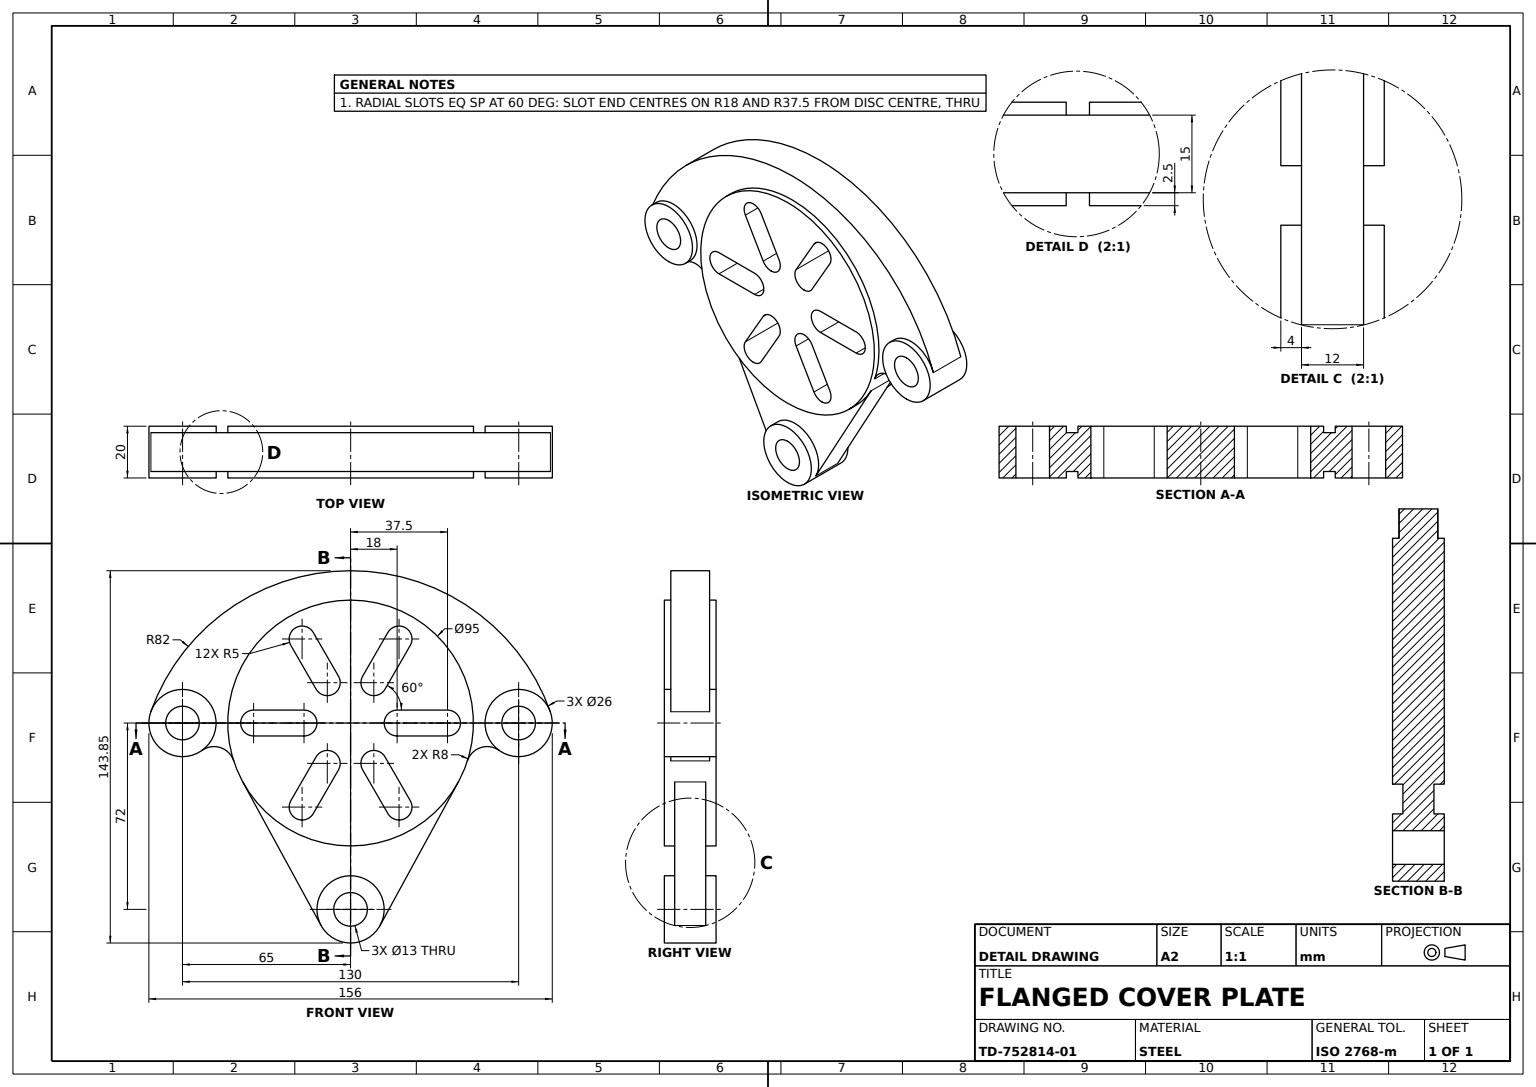
solid
v1 (-14.4198729811,0,-34.9759526419)
v2 (-14.4198729811,20,-34.9759526419)
e1 v1 v2 LINE
v3 (-23.0801270189,20,-29.9759526419)
e2 v2 v3 CIRCLE(AX(P(-18.75,20,-32.4759526419),D(0,1,0),D(0,0,1)),5)
v4 (-23.0801270189,0,-29.9759526419)
e3 v4 v3 LINE
e4 v1 v4 CIRCLE(AX(P(-18.75,0,-32.4759526419),D(0,1,0),D(0,0,1)),5)
face CYL(AX(P(-18.75,0,-32.4759526419),D(0,1,0),D(0,0,1)),5) rev [e1 e2 -e3 -e4]
v5 (9,0,-10.5884572681)
v6 (9,20,-10.5884572681)
e5 v5 v6 LINE
v7 (4.6698729811,0,-18.0884572681)
e6 v7 v5 CIRCLE(AX(P(9,0,-15.5884572681),D(0,1,0),D(0,0,1)),5)
v8 (4.6698729811,20,-18.0884572681)
e7 v7 v8 LINE
e8 v8 v6 CIRCLE(AX(P(9,20,-15.5884572681),D(0,1,0),D(0,0,1)),5)
face CYL(AX(P(9,0,-15.5884572681),D(0,1,0),D(0,0,1)),5) rev [-e5 -e6 e7 e8]
v9 (77.2463768116,2.5,-4.3619095576)
v10 (0,2.5,-58.8483261944)
e9 v9 v10 CIRCLE(AX(P(0,2.5,23.1516738056),D(0,1,0),D(0,0,-1)),82)
v11 (0,17.5,-58.8483261944)
e10 v11 v10 LINE
v12 (77.2463768116,17.5,-4.3619095576)
e11 v12 v11 CIRCLE(AX(P(0,17.5,23.1516738056),D(0,1,0),D(0,0,-1)),82)
e12 v12 v9 LINE
face CYL(AX(P(0,17.5,23.1516738056),D(0,-1,0),D(0,0,-1)),82) [e9 -e10 -e11 e12]
v13 (13.3301270189,0,13.0884572681)
v14 (13.3301270189,20,13.0884572681)
e13 v13 v14 LINE
v15 (23.0801270189,0,29.9759526419)
e14 v13 v15 LINE
v16 (23.0801270189,20,29.9759526419)
e15 v15 v16 LINE
e16 v14 v16 LINE
face PLANE(AX(P(4.3301270189,0,-2.5),D(-0.8660254038,0,0.5),D(0.5,0,0.8660254038))) [-e13 e14 e15 -e16]
v17 (65,20,6.5)
v18 (65,0,6.5)
e17 v17 v18 LINE
v19 (65,20,-6.5)
e18 v17 v19 CIRCLE(AX(P(65,20,0),D(0,1,0),D(0,0,1)),6.5)
v20 (65,0,-6.5)
e19 v19 v20 LINE
e20 v18 v20 CIRCLE(AX(P(65,0,0),D(0,1,0),D(0,0,1)),6.5)
face CYL(AX(P(65,20,0),D(0,-1,0),D(0,0,-1)),6.5) rev [-e17 e18 e19 -e20]
v21 (-13.3301270189,20,-13.0884572681)
e21 v21 v3 LINE
v22 (-13.3301270189,0,-13.0884572681)
e22 v22 v21 LINE
e23 v22 v4 LINE
face PLANE(AX(P(-4.3301270189,0,2.5),D(0.8660254038,0,-0.5),D(-0.5,0,-0.8660254038))) [-e21 -e22 e23 e3]
v23 (-52.8019230769,17.5,9.0940609388)
v24 (-52.8019230769,2.5,9.0940609388)
e24 v23 v24 LINE
v25 (-45.1908350658,2.5,14.6300521548)
e25 v24 v25 CIRCLE(AX(P(-52.8019230769,2.5,17.0940609388),D(0,-1,0),D(0,0,-1)),8)
v26 (-45.1908350658,17.5,14.6300521548)
e26 v26 v25 LINE
e27 v23 v26 CIRCLE(AX(P(-52.8019230769,17.5,17.0940609388),D(0,-1,0),D(0,0,-1)),8)
face CYL(AX(P(-52.8019230769,17.5,17.0940609388),D(0,-1,0),D(0,0,-1)),8) rev [e24 e25 -e26 -e27]
v27 (0,16,59)
v28 (11.4104111512,16,78.2291666667)
e28 v27 v28 CIRCLE(AX(P(0,16,72),D(0,-1,0),D(0,0,1)),13)
v29 (41.6918868985,16,22.7604166667)
e29 v28 v29 LINE
v30 (0,16,47.5)
e30 v29 v30 CIRCLE(AX(P(0,16,0),D(0,-1,0),D(0,0,1)),47.5)
v31 (-41.6918868985,16,22.7604166667)
e31 v30 v31 CIRCLE(AX(P(0,16,0),D(0,-1,0),D(0,0,1)),47.5)
v32 (-11.4104111512,16,78.2291666667)
e32 v31 v32 LINE
e33 v32 v27 CIRCLE(AX(P(0,16,72),D(0,-1,0),D(0,0,1)),13)
face PLANE(AX(P(0,16,0),D(0,1,0),D(0,0,1))) [e28 e29 e30 e31 e32 e33]
v33 (18,0,5)
v34 (37.5,0,5)
e34 v33 v34 LINE
v35 (18,20,5)
e35 v33 v35 LINE
v36 (37.5,20,5)
e36 v35 v36 LINE
e37 v34 v36 LINE
face PLANE(AX(P(0,0,5),D(0,0,1),D(1,0,0))) rev [-e34 e35 e36 -e37]
v37 (-57.4488095238,17.5,10.582037724)
v38 (-57.4488095238,2.5,10.582037724)
e38 v37 v38 LINE
e39 v38 v24 CIRCLE(AX(P(-52.8019230769,2.5,17.0940609388),D(0,-1,0),D(0,0,-1)),8)
e40 v37 v23 CIRCLE(AX(P(-52.8019230769,17.5,17.0940609388),D(0,-1,0),D(0,0,-1)),8)
face CYL(AX(P(-52.8019230769,17.5,17.0940609388),D(0,-1,0),D(0,0,-1)),8) rev [e38 e39 -e24 -e40]
v39 (-65,20,-6.5)
v40 (-65,0,-6.5)
e41 v39 v40 LINE
v41 (-65,0,6.5)
e42 v41 v40 CIRCLE(AX(P(-65,0,0),D(0,1,0),D(0,0,1)),6.5)
v42 (-65,20,6.5)
e43 v42 v41 LINE
e44 v42 v39 CIRCLE(AX(P(-65,20,0),D(0,1,0),D(0,0,1)),6.5)
face CYL(AX(P(-65,20,0),D(0,-1,0),D(0,0,-1)),6.5) rev [e41 -e42 -e43 e44]
v43 (4.6698729811,20,18.0884572681)
e45 v14 v43 CIRCLE(AX(P(9,20,15.5884572681),D(0,1,0),D(0,0,1)),5)
v44 (4.6698729811,0,18.0884572681)
e46 v44 v43 LINE
e47 v13 v44 CIRCLE(AX(P(9,0,15.5884572681),D(0,1,0),D(0,0,1)),5)
face CYL(AX(P(9,0,15.5884572681),D(0,1,0),D(0,0,1)),5) rev [e13 e45 -e46 -e47]
v45 (18,0,-5)
e48 v45 v33 CIRCLE(AX(P(18,0,0),D(0,1,0),D(0,0,1)),5)
v46 (18,20,-5)
e49 v45 v46 LINE
e50 v46 v35 CIRCLE(AX(P(18,20,0),D(0,1,0),D(0,0,1)),5)
face CYL(AX(P(18,0,0),D(0,1,0),D(0,0,1)),5) rev [-e48 e49 e50 -e35]
v47 (-4.6698729811,0,18.0884572681)
v48 (-13.3301270189,0,13.0884572681)
e51 v47 v48 CIRCLE(AX(P(-9,0,15.5884572681),D(0,1,0),D(0,0,1)),5)
v49 (-4.6698729811,20,18.0884572681)
e52 v47 v49 LINE
v50 (-13.3301270189,20,13.0884572681)
e53 v49 v50 CIRCLE(AX(P(-9,20,15.5884572681),D(0,1,0),D(0,0,1)),5)
e54 v48 v50 LINE
face CYL(AX(P(-9,0,15.5884572681),D(0,1,0),D(0,0,1)),5) rev [-e51 e52 e53 -e54]
v51 (65,17.5,-13)
e55 v12 v51 CIRCLE(AX(P(65,17.5,0),D(0,1,0),D(0,0,-1)),13)
v52 (65,20,-13)
e56 v52 v51 LINE
v53 (65,20,13)
e57 v53 v52 CIRCLE(AX(P(65,20,0),D(0,1,0),D(0,0,1)),13)
v54 (65,0,13)
e58 v53 v54 LINE
v55 (65,0,-13)
e59 v54 v55 CIRCLE(AX(P(65,0,0),D(0,1,0),D(0,0,1)),13)
v56 (65,2.5,-13)
e60 v56 v55 LINE
e61 v9 v56 CIRCLE(AX(P(65,2.5,0),D(0,1,0),D(0,0,-1)),13)
face CYL(AX(P(65,17.5,0),D(0,-1,0),D(0,0,-1)),13) [e55 -e56 -e57 e58 e59 -e60 -e61 -e12]
e62 v52 v53 CIRCLE(AX(P(65,20,0),D(0,1,0),D(0,0,1)),13)
v57 (57.4488095238,17.5,10.582037724)
e63 v51 v57 CIRCLE(AX(P(65,17.5,0),D(0,1,0),D(0,0,-1)),13)
v58 (57.4488095238,2.5,10.582037724)
e64 v57 v58 LINE
e65 v56 v58 CIRCLE(AX(P(65,2.5,0),D(0,1,0),D(0,0,-1)),13)
e66 v55 v54 CIRCLE(AX(P(65,0,0),D(0,1,0),D(0,0,1)),13)
face CYL(AX(P(65,17.5,0),D(0,-1,0),D(0,0,-1)),13) [-e58 -e62 e56 e63 e64 -e65 e60 e66]
v59 (0,4,59)
v60 (11.4104111512,4,78.2291666667)
e67 v59 v60 CIRCLE(AX(P(0,4,72),D(0,-1,0),D(0,0,1)),13)
v61 (-11.4104111512,4,78.2291666667)
e68 v61 v59 CIRCLE(AX(P(0,4,72),D(0,-1,0),D(0,0,1)),13)
v62 (-41.6918868985,4,22.7604166667)
e69 v62 v61 LINE
v63 (0,4,47.5)
e70 v63 v62 CIRCLE(AX(P(0,4,0),D(0,-1,0),D(0,0,1)),47.5)
v64 (41.6918868985,4,22.7604166667)
e71 v64 v63 CIRCLE(AX(P(0,4,0),D(0,-1,0),D(0,0,1)),47.5)
e72 v60 v64 LINE
face PLANE(AX(P(0,4,0),D(0,1,0),D(0,0,1))) rev [-e67 -e68 -e69 -e70 -e71 -e72]
v65 (13.3301270189,20,-13.0884572681)
e73 v6 v65 CIRCLE(AX(P(9,20,-15.5884572681),D(0,1,0),D(0,0,1)),5)
v66 (13.3301270189,0,-13.0884572681)
e74 v66 v65 LINE
e75 v5 v66 CIRCLE(AX(P(9,0,-15.5884572681),D(0,1,0),D(0,0,1)),5)
face CYL(AX(P(9,0,-15.5884572681),D(0,1,0),D(0,0,1)),5) rev [e73 -e74 -e75 e5]
v67 (-14.4198729811,20,34.9759526419)
e76 v49 v67 LINE
v68 (-14.4198729811,0,34.9759526419)
e77 v47 v68 LINE
e78 v68 v67 LINE
face PLANE(AX(P(4.3301270189,0,2.5),D(-0.8660254038,0,-0.5),D(-0.5,0,0.8660254038))) [-e76 -e52 e77 e78]
e79 v29 v64 LINE
e80 v28 v60 LINE
face PLANE(AX(P(41.6918868985,16,22.7604166667),D(-0.8777239347,0,-0.4791666667),D(-0.4791666667,0,0.8777239347))) rev [-e79 -e29 e80 e72]
e81 v19 v17 CIRCLE(AX(P(65,20,0),D(0,1,0),D(0,0,1)),6.5)
face PLANE(AX(P(65,20,0),D(0,1,0),D(0,0,1))) [e62 e57] [-e18 -e81]
v69 (-18.75,20,37.4759526419)
e82 v69 v67 CIRCLE(AX(P(-18.75,20,32.4759526419),D(0,1,0),D(0,0,1)),5)
v70 (-18.75,0,37.4759526419)
e83 v70 v68 CIRCLE(AX(P(-18.75,0,32.4759526419),D(0,1,0),D(0,0,1)),5)
e84 v70 v69 LINE
face CYL(AX(P(-18.75,0,32.4759526419),D(0,1,0),D(0,0,1)),5) rev [e82 -e78 -e83 e84]
v71 (0,20,85)
v72 (0,20,59)
e85 v71 v72 CIRCLE(AX(P(0,20,72),D(0,1,0),D(0,0,1)),13)
e86 v72 v71 CIRCLE(AX(P(0,20,72),D(0,1,0),D(0,0,1)),13)
v73 (0,20,65.5)
v74 (0,20,78.5)
e87 v73 v74 CIRCLE(AX(P(0,20,72),D(0,1,0),D(0,0,1)),6.5)
e88 v74 v73 CIRCLE(AX(P(0,20,72),D(0,1,0),D(0,0,1)),6.5)
face PLANE(AX(P(0,20,72),D(0,1,0),D(0,0,1))) [e85 e86] [-e87 -e88]
v75 (0,0,85)
v76 (0,0,59)
e89 v75 v76 CIRCLE(AX(P(0,0,72),D(0,1,0),D(0,0,1)),13)
e90 v76 v75 CIRCLE(AX(P(0,0,72),D(0,1,0),D(0,0,1)),13)
v77 (0,0,78.5)
v78 (0,0,65.5)
e91 v77 v78 CIRCLE(AX(P(0,0,72),D(0,1,0),D(0,0,1)),6.5)
e92 v78 v77 CIRCLE(AX(P(0,0,72),D(0,1,0),D(0,0,1)),6.5)
face PLANE(AX(P(0,0,72),D(0,1,0),D(0,0,1))) rev [-e89 -e90] [e91 e92]
v79 (23.0801270189,0,-29.9759526419)
v80 (14.4198729811,0,-34.9759526419)
e93 v79 v80 CIRCLE(AX(P(18.75,0,-32.4759526419),D(0,1,0),D(0,0,1)),5)
v81 (23.0801270189,20,-29.9759526419)
e94 v79 v81 LINE
v82 (14.4198729811,20,-34.9759526419)
e95 v81 v82 CIRCLE(AX(P(18.75,20,-32.4759526419),D(0,1,0),D(0,0,1)),5)
e96 v80 v82 LINE
face CYL(AX(P(18.75,0,-32.4759526419),D(0,1,0),D(0,0,1)),5) rev [-e93 e94 e95 -e96]
e97 v7 v80 LINE
e98 v8 v82 LINE
face PLANE(AX(P(-4.3301270189,0,-2.5),D(0.8660254038,0,0.5),D(0.5,0,-0.8660254038))) [e97 e96 -e98 -e7]
v83 (-23.0801270189,0,29.9759526419)
v84 (-23.0801270189,20,29.9759526419)
e99 v83 v84 LINE
e100 v84 v69 CIRCLE(AX(P(-18.75,20,32.4759526419),D(0,1,0),D(0,0,1)),5)
e101 v83 v70 CIRCLE(AX(P(-18.75,0,32.4759526419),D(0,1,0),D(0,0,1)),5)
face CYL(AX(P(-18.75,0,32.4759526419),D(0,1,0),D(0,0,1)),5) rev [e99 e100 -e84 -e101]
e102 v78 v73 LINE
e103 v77 v74 LINE
face CYL(AX(P(0,0,72),D(0,1,0),D(0,0,1)),6.5) rev [e102 e87 -e103 -e92]
v85 (-77.2463768116,17.5,-4.3619095576)
e104 v11 v85 CIRCLE(AX(P(0,17.5,23.1516738056),D(0,1,0),D(0,0,-1)),82)
v86 (-65,17.5,-13)
e105 v86 v85 CIRCLE(AX(P(-65,17.5,0),D(0,1,0),D(0,0,-1)),13)
e106 v37 v86 CIRCLE(AX(P(-65,17.5,0),D(0,1,0),D(0,0,-1)),13)
v87 (0,17.5,-47.5)
e107 v26 v87 CIRCLE(AX(P(0,17.5,0),D(0,-1,0),D(0,0,-1)),47.5)
v88 (45.1908350658,17.5,14.6300521548)
e108 v87 v88 CIRCLE(AX(P(0,17.5,0),D(0,-1,0),D(0,0,-1)),47.5)
v89 (52.8019230769,17.5,9.0940609388)
e109 v88 v89 CIRCLE(AX(P(52.8019230769,17.5,17.0940609388),D(0,-1,0),D(0,0,-1)),8)
e110 v89 v57 CIRCLE(AX(P(52.8019230769,17.5,17.0940609388),D(0,-1,0),D(0,0,-1)),8)
face PLANE(AX(P(32.5,17.5,11.5758369028),D(0,-1,0),D(0,0,-1))) rev [-e63 -e55 e11 e104 -e105 -e106 e40 e27 e107 e108 e109 e110]
v90 (-9,20,-10.5884572681)
v91 (-4.6698729811,20,-18.0884572681)
e111 v90 v91 CIRCLE(AX(P(-9,20,-15.5884572681),D(0,1,0),D(0,0,1)),5)
v92 (-4.6698729811,0,-18.0884572681)
e112 v92 v91 LINE
v93 (-9,0,-10.5884572681)
e113 v93 v92 CIRCLE(AX(P(-9,0,-15.5884572681),D(0,1,0),D(0,0,1)),5)
e114 v93 v90 LINE
face CYL(AX(P(-9,0,-15.5884572681),D(0,1,0),D(0,0,1)),5) rev [e111 -e112 -e113 e114]
v94 (18.75,0,37.4759526419)
v95 (18.75,20,37.4759526419)
e115 v94 v95 LINE
e116 v95 v16 CIRCLE(AX(P(18.75,20,32.4759526419),D(0,1,0),D(0,0,1)),5)
e117 v94 v15 CIRCLE(AX(P(18.75,0,32.4759526419),D(0,1,0),D(0,0,1)),5)
face CYL(AX(P(18.75,0,32.4759526419),D(0,1,0),D(0,0,1)),5) rev [e115 e116 -e15 -e117]
v96 (52.8019230769,2.5,9.0940609388)
e118 v89 v96 LINE
e119 v96 v58 CIRCLE(AX(P(52.8019230769,2.5,17.0940609388),D(0,-1,0),D(0,0,-1)),8)
face CYL(AX(P(52.8019230769,17.5,17.0940609388),D(0,-1,0),D(0,0,-1)),8) rev [e118 e119 -e64 -e110]
v97 (14.4198729811,0,34.9759526419)
v98 (14.4198729811,20,34.9759526419)
e120 v97 v98 LINE
e121 v98 v95 CIRCLE(AX(P(18.75,20,32.4759526419),D(0,1,0),D(0,0,1)),5)
e122 v97 v94 CIRCLE(AX(P(18.75,0,32.4759526419),D(0,1,0),D(0,0,1)),5)
face CYL(AX(P(18.75,0,32.4759526419),D(0,1,0),D(0,0,1)),5) rev [e120 e121 -e115 -e122]
v99 (-18,0,5)
v100 (-18,20,5)
e123 v99 v100 LINE
v101 (-18,20,-5)
e124 v100 v101 CIRCLE(AX(P(-18,20,0),D(0,1,0),D(0,0,1)),5)
v102 (-18,0,-5)
e125 v102 v101 LINE
e126 v99 v102 CIRCLE(AX(P(-18,0,0),D(0,1,0),D(0,0,1)),5)
face CYL(AX(P(-18,0,0),D(0,1,0),D(0,0,1)),5) rev [e123 e124 -e125 -e126]
e127 v31 v62 LINE
e128 v32 v61 LINE
face PLANE(AX(P(-41.6918868985,16,22.7604166667),D(0.8777239347,0,-0.4791666667),D(-0.4791666667,0,-0.8777239347))) rev [e127 e69 -e128 -e32]
e129 v50 v84 LINE
e130 v48 v83 LINE
face PLANE(AX(P(-4.3301270189,0,-2.5),D(-0.8660254038,0,-0.5),D(-0.5,0,0.8660254038))) rev [e129 -e99 -e130 e54]
v103 (37.5,20,-5)
e131 v46 v103 LINE
e132 v36 v103 CIRCLE(AX(P(37.5,20,0),D(0,1,0),D(0,0,1)),5)
v104 (0,20,47.5)
v105 (0,20,-47.5)
e133 v104 v105 CIRCLE(AX(P(0,20,0),D(0,1,0),D(0,0,1)),47.5)
e134 v105 v104 CIRCLE(AX(P(0,20,0),D(0,1,0),D(0,0,1)),47.5)
e135 v65 v81 LINE
e136 v21 v90 CIRCLE(AX(P(-9,20,-15.5884572681),D(0,1,0),D(0,0,1)),5)
e137 v91 v2 LINE
v106 (-37.5,20,5)
e138 v100 v106 LINE
v107 (-37.5,20,-5)
e139 v107 v106 CIRCLE(AX(P(-37.5,20,0),D(0,1,0),D(0,0,1)),5)
e140 v101 v107 LINE
e141 v43 v98 LINE
face PLANE(AX(P(0,20,0),D(0,1,0),D(0,0,1))) [e131 -e132 -e36 -e50] [e133 e134] [-e73 -e8 e98 -e95 -e135] [-e100 -e129 -e53 e76 -e82] [-e136 e21 -e2 -e137 -e111] [-e124 e138 -e139 -e140] [-e121 -e141 -e45 e16 -e116]
e142 v20 v18 CIRCLE(AX(P(65,0,0),D(0,1,0),D(0,0,1)),6.5)
face PLANE(AX(P(65,0,0),D(0,1,0),D(0,0,1))) rev [-e59 -e66] [e20 e142]
e143 v72 v27 LINE
e144 v71 v75 LINE
e145 v59 v76 LINE
face CYL(AX(P(0,16,72),D(0,-1,0),D(0,0,-1)),13) [-e28 -e143 -e85 e144 e89 -e145 e67 -e80]
v108 (37.5,0,-5)
e146 v45 v108 LINE
e147 v108 v103 LINE
face PLANE(AX(P(0,0,-5),D(0,0,1),D(1,0,0))) [e146 e147 -e131 -e49]
v109 (-77.2463768116,2.5,-4.3619095576)
e148 v10 v109 CIRCLE(AX(P(0,2.5,23.1516738056),D(0,1,0),D(0,0,-1)),82)
v110 (45.1908350658,2.5,14.6300521548)
e149 v110 v96 CIRCLE(AX(P(52.8019230769,2.5,17.0940609388),D(0,-1,0),D(0,0,-1)),8)
v111 (0,2.5,-47.5)
e150 v111 v110 CIRCLE(AX(P(0,2.5,0),D(0,-1,0),D(0,0,-1)),47.5)
e151 v25 v111 CIRCLE(AX(P(0,2.5,0),D(0,-1,0),D(0,0,-1)),47.5)
v112 (-65,2.5,-13)
e152 v38 v112 CIRCLE(AX(P(-65,2.5,0),D(0,1,0),D(0,0,-1)),13)
e153 v112 v109 CIRCLE(AX(P(-65,2.5,0),D(0,1,0),D(0,0,-1)),13)
face PLANE(AX(P(32.5,2.5,11.5758369028),D(0,-1,0),D(0,0,-1))) [-e148 -e9 e61 e65 -e119 -e149 -e150 -e151 -e25 -e39 e152 e153]
v113 (-65,20,-13)
v114 (-65,20,13)
e154 v113 v114 CIRCLE(AX(P(-65,20,0),D(0,1,0),D(0,0,1)),13)
e155 v113 v86 LINE
e156 v85 v109 LINE
v115 (-65,0,-13)
e157 v112 v115 LINE
v116 (-65,0,13)
e158 v115 v116 CIRCLE(AX(P(-65,0,0),D(0,1,0),D(0,0,1)),13)
e159 v114 v116 LINE
face CYL(AX(P(-65,17.5,0),D(0,-1,0),D(0,0,-1)),13) [-e154 e155 e105 e156 -e153 e157 e158 -e159]
face CYL(AX(P(0,17.5,23.1516738056),D(0,-1,0),D(0,0,-1)),82) [-e104 e10 e148 -e156]
e160 v34 v108 CIRCLE(AX(P(37.5,0,0),D(0,1,0),D(0,0,1)),5)
face CYL(AX(P(37.5,0,0),D(0,1,0),D(0,0,1)),5) rev [-e147 -e160 e37 e132]
e161 v104 v30 LINE
e162 v105 v87 LINE
v117 (0,0,-47.5)
e163 v111 v117 LINE
v118 (0,0,47.5)
e164 v117 v118 CIRCLE(AX(P(0,0,0),D(0,1,0),D(0,0,1)),47.5)
e165 v63 v118 LINE
face CYL(AX(P(0,20,0),D(0,-1,0),D(0,0,-1)),47.5) [-e31 -e161 -e134 e162 -e107 e26 e151 e163 e164 -e165 e70 -e127]
e166 v114 v113 CIRCLE(AX(P(-65,20,0),D(0,1,0),D(0,0,1)),13)
e167 v116 v115 CIRCLE(AX(P(-65,0,0),D(0,1,0),D(0,0,1)),13)
face CYL(AX(P(-65,17.5,0),D(0,-1,0),D(0,0,-1)),13) [e106 -e155 -e166 e159 e167 -e157 -e152 -e38]
e168 v66 v79 LINE
face PLANE(AX(P(4.3301270189,0,2.5),D(0.8660254038,0,0.5),D(0.5,0,-0.8660254038))) rev [e135 -e94 -e168 e74]
e169 v40 v41 CIRCLE(AX(P(-65,0,0),D(0,1,0),D(0,0,1)),6.5)
face PLANE(AX(P(-65,0,0),D(0,1,0),D(0,0,1))) rev [-e167 -e158] [e169 e42]
e170 v39 v42 CIRCLE(AX(P(-65,20,0),D(0,1,0),D(0,0,1)),6.5)
face CYL(AX(P(-65,20,0),D(0,-1,0),D(0,0,-1)),6.5) rev [-e169 -e41 e170 e43]
face CYL(AX(P(0,0,72),D(0,1,0),D(0,0,1)),6.5) rev [e103 e88 -e102 -e91]
e171 v44 v97 LINE
face PLANE(AX(P(-4.3301270189,0,2.5),D(-0.8660254038,0,0.5),D(0.5,0,0.8660254038))) rev [-e120 -e171 e46 e141]
e172 v118 v117 CIRCLE(AX(P(0,0,0),D(0,1,0),D(0,0,1)),47.5)
e173 v88 v110 LINE
face CYL(AX(P(0,20,0),D(0,-1,0),D(0,0,-1)),47.5) [e161 -e30 e79 e71 e165 e172 -e163 e150 -e173 -e108 -e162 -e133]
face CYL(AX(P(65,20,0),D(0,-1,0),D(0,0,-1)),6.5) rev [e81 e17 -e142 -e19]
e174 v92 v1 LINE
face PLANE(AX(P(4.3301270189,0,-2.5),D(0.8660254038,0,-0.5),D(-0.5,0,-0.8660254038))) rev [-e1 -e174 e112 e137]
v119 (-37.5,0,-5)
e175 v119 v107 LINE
e176 v102 v119 LINE
face PLANE(AX(P(0,0,-5),D(0,0,-1),D(-1,0,0))) rev [-e175 -e176 e125 e140]
e177 v22 v93 CIRCLE(AX(P(-9,0,-15.5884572681),D(0,1,0),D(0,0,1)),5)
face CYL(AX(P(-9,0,-15.5884572681),D(0,1,0),D(0,0,1)),5) rev [-e114 -e177 e22 e136]
face CYL(AX(P(52.8019230769,17.5,17.0940609388),D(0,-1,0),D(0,0,-1)),8) rev [-e118 -e109 e173 e149]
v120 (-37.5,0,5)
e178 v120 v106 LINE
e179 v119 v120 CIRCLE(AX(P(-37.5,0,0),D(0,1,0),D(0,0,1)),5)
face CYL(AX(P(-37.5,0,0),D(0,1,0),D(0,0,1)),5) rev [e175 e139 -e178 -e179]
e180 v99 v120 LINE
face PLANE(AX(P(0,0,0),D(0,1,0),D(0,0,1))) rev [e160 -e146 e48 e34] [-e97 e6 e75 e168 e93] [e117 -e14 e47 e171 e122] [e83 -e77 e51 e130 e101] [e126 e176 e179 -e180] [-e164 -e172] [e174 e4 -e23 e177 e113]
face CYL(AX(P(0,16,72),D(0,-1,0),D(0,0,-1)),13) [e90 -e144 -e86 e143 -e33 e128 e68 e145]
face PLANE(AX(P(-65,20,0),D(0,1,0),D(0,0,1))) [e154 e166] [-e170 -e44]
face PLANE(AX(P(0,0,5),D(0,0,-1),D(-1,0,0))) [e180 e178 -e138 -e123]
